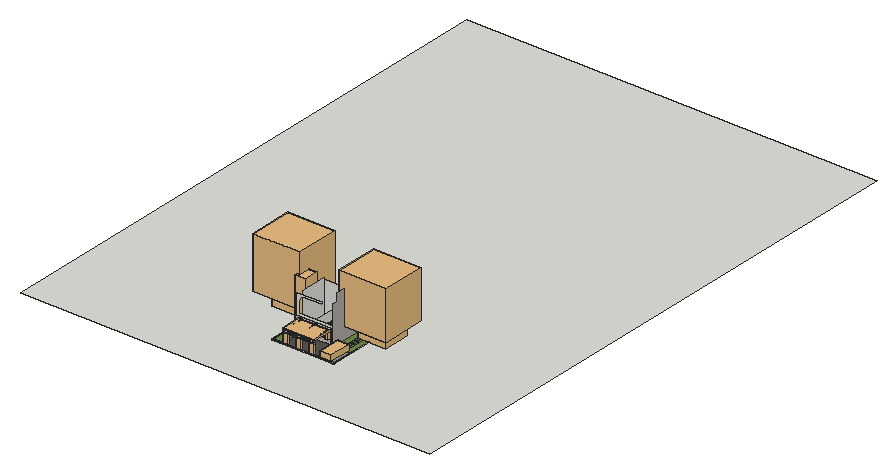
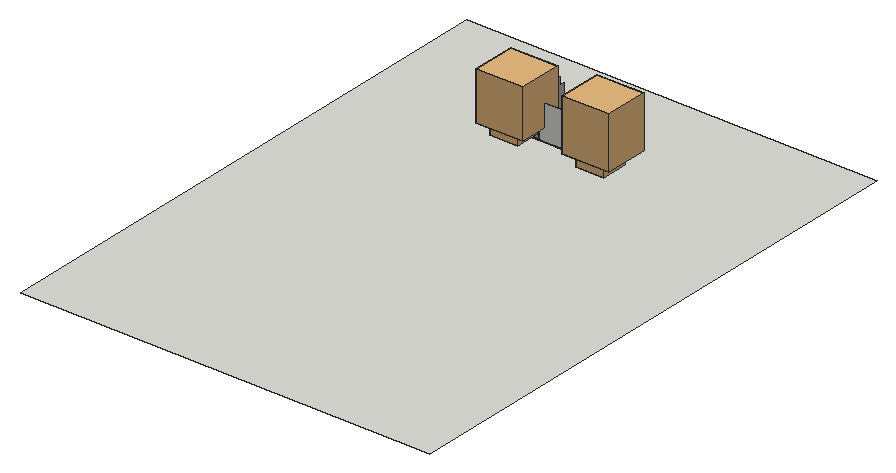
# SketchUp Ruby script. Lengths in inches.
U = 1.inch
M = Sketchup.active_model
def pt(a) = Geom::Point3d.new(a.map { |v| v * U })
def face(e, loops, mat)
  f = e.add_face(loops[0].map { |a| pt(a) })
  loops[1..].each { |l| e.add_face(l.map { |a| pt(a) }).erase! }
  f.material = f.back_material = mat if mat
  f
end
# faces: each face lists its corners as indices into pts; further lists are holes
def faces(e, pts, list, mat = nil) = list.each { |f| face(e, (f[0].is_a?(Array) ? f : [f]).map { |l| l.map { |i| pts[i] } }, mat) }
# xy, xz, yz: faces in a plane at the given z, y or x. An outline is a flat list of corners, or four numbers for a rectangle; further outlines are holes
def ring(l) = l.size == 4 ? [[l[0], l[1]], [l[2], l[1]], [l[2], l[3]], [l[0], l[3]]] : l.each_slice(2).to_a
def flat(e, list, mat, &to3) = list.each { |f| face(e, (f[0].is_a?(Array) ? f : [f]).map { |l| ring(l).map { |u, v| to3.(u, v) } }, mat) }
def xy(e, z, list, mat = nil) = flat(e, list, mat) { |x, y| [x, y, z] }
def xz(e, y, list, mat = nil) = flat(e, list, mat) { |x, z| [x, y, z] }
def yz(e, x, list, mat = nil) = flat(e, list, mat) { |y, z| [x, y, z] }
def lines(e, pts, list) = list.each { |a, b| e.add_line(pt(pts[a]), pt(pts[b])) }
# prism: a flat outline (further loops are holes) pulled along v
def prism(e, loops, v, mat = nil)
  f = face(e, loops, mat); d = Geom::Vector3d.new(v.map { |x| x * U })
  f.pushpull(f.normal.samedirection?(d) ? d.length : -d.length)
end
def box(e, o, s, mat = nil) = prism(e, [[o, [o[0] + s[0], o[1], o[2]], [o[0] + s[0], o[1] + s[1], o[2]], [o[0], o[1] + s[1], o[2]]]], [0, 0, s[2]], mat)
def at(x, y, z, deg = 0) = Geom::Transformation.translation(pt([x, y, z])) * Geom::Transformation.rotation(ORIGIN, Z_AXIS, deg.degrees)
def axes(o, x, y, z) = Geom::Transformation.new([*x, 0, *y, 0, *z, 0, *pt(o).to_a, 1])
def part(name) = M.definitions.add(name)
# library, detail: a bought-in or finely detailed component or shape, given as its bounding box
def library(name, o, s) = part(name).tap { |d| box(d.entities, o, s) }
def detail(e, o, s) = box(e.add_group.entities, o, s)
def put(e, d, t, mat = nil) = e.add_instance(d, t).tap { |i| i.material = mat if mat }
def group(e, t, mat = nil) = e.add_group.tap { |g| g.transformation = t; g.material = mat if mat }.entities
root = M.entities
M.materials.add("AM113_062_Tilia").color = [58, 81, 37]
M.materials.add("AM113_062_Tilia_Bark").color = [88, 85, 72]
M.materials.add("Grass D 200cm").color = [112, 140, 73]
M.materials.add("Grass D 200cm\#1").color = [112, 140, 73]
M.materials.add("Pavement Concrete 03 300cm").color = [155, 154, 151]
M.materials.add("Pavement Rock Tiles 19-79 250cm").color = [91, 85, 85]
M.materials.add("Sandstone 150cm").color = [161, 146, 124]
M.materials.add("Stone D 150cm").color = [179, 173, 168]
M.materials.add("Tiles L01 200cm").color = [179, 171, 162]
M.materials.add("Wall Paint Fine Grain 01 Yellow 100cm").color = [244, 233, 200]
M.materials.add("Wood066_2K_Color").color = [89, 51, 19]
M.materials.add("[Color M05]").color = [114, 114, 114]
M.materials.add("[Color M07]1").color = [58, 58, 58]
M.materials.add("[Color M08]").color = [30, 30, 30]
M.materials.add("[Tile_Various_Tan]").color = [214, 196, 169]
c1 = part("Group3\#2")
p = [[646.26,365.625,0],[646.26,367.5625,0],[646.26,485.6875,58.75],[646.26,523.125,58.75],[725.07,523.125,58.75],[725.07,485.6875,58.75],
  [725.07,367.5625,117.5],[725.07,355.75,117.5],[681.76,365.625,0],[681.76,367.5625,0],[681.76,485.6875,58.75],[681.76,487.625,58.75],
  [689.57,487.625,58.75],[689.57,485.6875,58.75],[689.57,367.5625,117.5],[689.57,355.75,117.5]]
lines(c1.entities,p,[[0,1],[1,2],[2,3],[3,4],[4,5],[5,6],[6,7],[8,9],[9,10],[10,11],[11,12],[12,13],
  [13,14],[14,15]])
c2 = part("Group2\#1")
xy(c2.entities,-3.9375,[[644.32,379.375,683.7,380.3]])
xy(c2.entities,0,[[644.32,367.5625,683.7,379.375]])
xy(c2.entities,5.875,[[644.32,379.375,683.7,391.1875]])
xy(c2.entities,11.75,[[644.32,391.1875,683.7,403]])
xy(c2.entities,17.625,[[644.32,403,683.7,414.8125]])
xy(c2.entities,23.5,[[644.32,414.8125,683.7,426.625]])
xy(c2.entities,29.375,[[644.32,426.625,683.7,438.4375]])
xy(c2.entities,35.25,[[644.32,438.4375,683.7,450.25]])
xy(c2.entities,41.125,[[644.32,450.25,683.7,462.0625]])
xy(c2.entities,47,[[644.32,462.0625,683.7,473.875]])
xy(c2.entities,52.875,[[644.32,473.875,683.7,485.6875]])
xy(c2.entities,54.8125,[[687.63,472.95,687.63,485.6875,683.7,485.6875,683.7,498.42,644.32,498.42,644.32,525.0625,727.01,525.0625,727.01,472.95]])
xy(c2.entities,58.75,[[687.63,473.875,727.01,473.875,727.01,525.0625,644.32,525.0625,644.32,485.6875,687.63,485.6875]])
xy(c2.entities,64.625,[[687.63,462.0625,727.01,473.875]])
xy(c2.entities,70.5,[[687.63,450.25,727.01,462.0625]])
xy(c2.entities,76.375,[[687.63,438.4375,727.01,450.25]])
xy(c2.entities,82.25,[[687.63,426.625,727.01,438.4375]])
xy(c2.entities,88.125,[[687.63,414.8125,727.01,426.625]])
xy(c2.entities,94,[[687.63,403,727.01,414.8125]])
xy(c2.entities,99.875,[[687.63,391.1875,727.01,403]])
xy(c2.entities,105.75,[[687.63,379.375,727.01,391.1875]])
xy(c2.entities,111.625,[[687.63,367.5625,727.01,379.375]])
xy(c2.entities,117.5,[[687.63,355.75,727.01,367.5625]])
xz(c2.entities,367.5625,[[687.63,111.625,727.01,117.5]])
xz(c2.entities,379.375,[[687.63,105.75,727.01,111.625]])
xz(c2.entities,379.375,[[644.32,0,683.7,5.875]],"[Color M05]")
xz(c2.entities,391.1875,[[687.63,99.875,727.01,105.75]])
xz(c2.entities,391.1875,[[644.32,5.875,683.7,11.75]],"[Color M05]")
xz(c2.entities,403,[[687.63,94,727.01,99.875]])
xz(c2.entities,403,[[644.32,11.75,683.7,17.625]],"[Color M05]")
xz(c2.entities,414.8125,[[687.63,88.125,727.01,94]])
xz(c2.entities,414.8125,[[644.32,17.625,683.7,23.5]],"[Color M05]")
xz(c2.entities,426.625,[[687.63,82.25,727.01,88.125]])
xz(c2.entities,426.625,[[644.32,23.5,683.7,29.375]],"[Color M05]")
xz(c2.entities,438.4375,[[687.63,76.375,727.01,82.25]])
xz(c2.entities,438.4375,[[644.32,29.375,683.7,35.25]],"[Color M05]")
xz(c2.entities,450.25,[[687.63,70.5,727.01,76.375]])
xz(c2.entities,450.25,[[644.32,35.25,683.7,41.125]],"[Color M05]")
xz(c2.entities,462.0625,[[687.63,64.625,727.01,70.5]])
xz(c2.entities,462.0625,[[644.32,41.125,683.7,47]],"[Color M05]")
xz(c2.entities,473.875,[[687.63,58.75,727.01,64.625]])
xz(c2.entities,473.875,[[644.32,47,683.7,52.875]],"[Color M05]")
xz(c2.entities,485.6875,[[644.32,52.875,683.7,58.75],[683.7,54.8125,687.63,58.75]],"[Color M05]")
xz(c2.entities,525.0625,[[644.32,54.8125,727.01,58.75]])
yz(c2.entities,644.32,[[379.375,-3.9375,379.375,5.875,391.1875,5.875,391.1875,11.75,403,11.75,403,17.625,414.8125,17.625,414.8125,23.5,426.625,23.5,426.625,29.375,438.4375,29.375,438.4375,35.25,450.25,35.25,450.25,41.125,462.0625,41.125,462.0625,47,473.875,47,473.875,52.875,485.6875,52.875,485.6875,58.75,525.0625,58.75,525.0625,54.8125,498.42,54.8125,380.3,-3.9375]])
yz(c2.entities,683.7,[[379.375,-3.9375,380.3,-3.9375,498.42,54.8125,485.6875,54.8125,485.6875,52.875,473.875,52.875,473.875,47,462.0625,47,462.0625,41.125,450.25,41.125,450.25,35.25,438.4375,35.25,438.4375,29.375,426.625,29.375,426.625,23.5,414.8125,23.5,414.8125,17.625,403,17.625,403,11.75,391.1875,11.75,391.1875,5.875,379.375,5.875]],"[Color M05]")
yz(c2.entities,687.63,[[472.95,54.8125,354.83,113.5625,355.75,113.5625,355.75,117.5,367.5625,117.5,367.5625,111.625,379.375,111.625,379.375,105.75,391.1875,105.75,391.1875,99.875,403,99.875,403,94,414.8125,94,414.8125,88.125,426.625,88.125,426.625,82.25,438.4375,82.25,438.4375,76.375,450.25,76.375,450.25,70.5,462.0625,70.5,462.0625,64.625,473.875,64.625,473.875,58.75,485.6875,58.75,485.6875,54.8125]],"[Color M05]")
yz(c2.entities,727.01,[[472.95,54.8125,525.0625,54.8125,525.0625,58.75,473.875,58.75,473.875,64.625,462.0625,64.625,462.0625,70.5,450.25,70.5,450.25,76.375,438.4375,76.375,438.4375,82.25,426.625,82.25,426.625,88.125,414.8125,88.125,414.8125,94,403,94,403,99.875,391.1875,99.875,391.1875,105.75,379.375,105.75,379.375,111.625,367.5625,111.625,367.5625,117.5,355.75,117.5,355.75,113.5625,354.83,113.5625]])
p = [[644.32,380.3,-3.9375],[644.32,498.42,54.8125],[683.7,498.42,54.8125],[683.7,380.3,-3.9375],[727.01,472.95,54.8125],[727.01,354.83,113.5625],
  [687.63,354.83,113.5625],[687.63,472.95,54.8125]]
faces(c2.entities,p,[[0,1,2,3]])
faces(c2.entities,p,[[4,5,6,7]],"[Color M05]")
put(c2.entities,c1,at(0,0,39.375))
c3 = library("Car 026",[-43.02,-94.05,-1.1],[86.04,187.94,58.68])
c4 = library("Plant",[-27.84,-31.84,-1.26],[68.28,70.82,154.38])
c5 = library("Agrupar\#1",[0,0,-45.2],[34.59,10.39,63.98])
c6 = library("AM113_062_Tilia_Defintion",[-350.67,-364.73,-2.58],[672.29,726.36,1000])
c7 = library("AM113_062_Tilia_Defintion1",[-524.84,-500,219.37],[933.41,1000,877.77])
c8 = part("Group4\#1")
put(c8.entities,c6,axes([0,0,0],[0.28109,0,0],[0,0.28109,0],[0,0,0.28109]),"AM113_062_Tilia_Bark")
put(c8.entities,c7,axes([0,0,0],[0.33697,0,0],[0,0.33697,0],[0,0,0.33697]),"AM113_062_Tilia")
c9 = library("Group4\#2",[-14.05,-12.91,-0.09],[26.62,27.13,73.11])
c10 = library("Agrupar\#17",[0,0,-45.2],[34.59,10.39,63.98])
c11 = library("Agrupar\#6",[0,0,-45.2],[34.59,10.39,63.98])
c12 = library("Shrub+_Grass",[-121.83,-22.34,0],[123.96,19.94,123.95])
c13 = part("Window (2)")
xy(c13.entities,31.72,[[-0.78,88.6,2.72,128.1]])
xy(c13.entities,34.95,[[-0.78,91.53,0.84,106.59],[0.84,91.53,1.05,97.58],[1.05,91.53,1.42,106.59],[1.42,91.53,2.72,106.59],[0.84,97.58,1.05,98.18],
  [0.84,98.18,1.05,106.59]])
xy(c13.entities,35.27,[[-0.78,110.09,0.97,125.14],[1.05,110.09,2.72,125.14]])
xy(c13.entities,58.35,[[2.72,108.74,3.8,109.74]])
xy(c13.entities,77.8125,[[-0.78,110.09,2.72,125.14],[0.97,110.09,1.05,125.14]])
xy(c13.entities,77.93,[[-0.78,91.53,0.84,106.59],[1.05,91.53,1.42,106.59],[1.42,91.53,2.72,106.59]])
xy(c13.entities,80.72,[[-0.78,88.6,2.72,128.1]])
xz(c13.entities,88.6,[[-0.78,31.72,2.72,80.72]])
xz(c13.entities,91.53,[[-0.78,34.95,0.84,77.93],[1.05,34.95,1.42,77.93],[1.42,34.95,2.72,77.93]])
xz(c13.entities,106.59,[[-0.78,34.95,0.84,77.93],[0.84,34.95,1.05,77.93],[0.84,34.95,2.72,77.93]])
xz(c13.entities,108.74,[[3.8,54.35,4.22,54.6,4.22,59.47,2.72,59.97,2.72,58.35,3.8,58.35]])
xz(c13.entities,109.74,[[3.8,54.35,3.8,58.35,2.72,58.35,2.72,59.97,4.22,59.47,4.22,54.6]])
xz(c13.entities,110.09,[[-0.78,35.27,0.97,77.8125],[1.05,35.27,2.72,77.8125]])
xz(c13.entities,125.14,[[-0.78,35.27,0.97,77.8125],[0.97,35.27,1.05,80.72],[1.05,35.27,2.72,77.8125]])
xz(c13.entities,128.1,[[-0.78,31.72,2.72,80.72]])
yz(c13.entities,-0.78,[[[88.6,31.72,128.1,80.72],[91.53,34.95,106.59,77.93],[110.09,35.27,125.14,77.8125]]])
yz(c13.entities,0.84,[[91.53,34.95,106.59,77.93]])
yz(c13.entities,0.97,[[110.09,35.27,125.14,77.8125]])
yz(c13.entities,1.05,[[91.53,34.95,106.59,77.93],[110.09,35.27,125.14,77.8125]])
yz(c13.entities,1.42,[[91.53,34.95,106.59,77.93]])
yz(c13.entities,2.72,[[[88.6,31.72,108.35,80.72],[91.53,34.95,106.59,77.93]],[[108.35,31.72,128.1,80.72],[110.09,35.27,125.14,77.8125],[108.74,58.35,109.74,59.97]]])
yz(c13.entities,3.8,[[108.74,54.35,109.74,58.35]])
yz(c13.entities,4.22,[[108.74,54.6,109.74,59.47]])
p = [[4.22,108.74,54.6],[3.8,108.74,54.35],[3.8,109.74,54.35],[4.22,109.74,54.6],[2.72,109.74,59.97],[2.72,108.74,59.97],
  [4.22,108.74,59.47],[4.22,109.74,59.47],[-0.78,86.4,89.94],[-0.78,86.44,89.94],[15.22,130.69,89.94],[15.22,130.65,89.94],
  [-0.78,86.44,28.19],[-0.78,86.4,28.19],[7.72,130.69,89.94],[7.72,130.65,89.94]]
faces(c13.entities,p,[[0,1,2,3],[4,5,6,7]])
lines(c13.entities,p,[[8,9],[10,11],[12,13],[14,15]])
c14 = library("Plant\#1",[-21.8,-11.875,0],[94.69,106.42,111.78])
c15 = part("Agrupar\#9")
prism(c15.entities,[[[223.78,9.67,1.43],[223.78,1.8,1.43],[-4.57,1.8,1.21],[-4.57,9.67,1.21]]],[-0.01,0,5.85])
p = [[218.86,1.8,0],[218.86,1.8,1.4],[218.86,9.68,1.4],[9.21,0.03,7.27],[9.18,0.03,7.27],[210,0,7.27],
  [209.97,0,7.27],[218.86,1.8,1.42],[9.21,0.03,7.27],[9.21,0,7.27],[210,9.67,1.4],[210,0.03,7.27],
  [209.97,0.03,7.27]]
lines(c15.entities,p,[[0,1],[1,2],[3,4],[5,6],[7,1],[8,9],[2,10],[11,5],[6,12],[12,11]])
c16 = part("Agrupar\#15")
prism(c16.entities,[[[7.43,175.26,4.98],[7.43,0,0],[7.43,0,13.77],[7.43,175.26,18.73]]],[-4.96,0,0])
p = [[3.57,19.55,0.34],[0.01,19.55,0.33],[0,11.68,0.33],[9.92,11.68,0.34]]
lines(c16.entities,p,[[0,1],[2,3]])
c17 = part("Agrupar\#11")
prism(c17.entities,[[[2.47,0,0],[2.47,175.26,4.98],[2.47,175.26,18.73],[2.47,0,13.77]]],[4.96,0,0])
p = [[3.57,19.55,0.34],[0.01,19.55,0.33],[6.3,204.91,6.81],[6.32,204.91,6.81],[0,11.68,0.33],[9.92,11.68,0.34]]
lines(c17.entities,p,[[0,1],[2,3],[4,5]])
c18 = library("Lugstar Premium LED 152 063",[-3.77,-3.75,-3.3125],[7.54,7.53,3.3125])
c19 = part("Tlon Cubo 860 Ceiling 152 005")
xy(c19.entities,-3.04,[[-16.54,-16.54,-16.54,16.54,16.54,-16.54],[16.54,-16.54,-16.54,16.54,16.54,16.54]])
xy(c19.entities,0,[[-16.93,-16.93,16.93,-16.93,-16.93,16.93],[16.93,-16.93,16.93,16.93,-16.93,16.93]])
xz(c19.entities,-16.93,[[-16.93,-3.79,16.93,-3.79,-16.93,0],[16.93,-3.79,16.93,0,-16.93,0]])
xz(c19.entities,-16.3,[[-16.3,-3.66,-16.3,-3.24,16.3,-3.24],[-16.3,-3.66,16.3,-3.24,16.3,-3.66]])
xz(c19.entities,16.3,[[-16.3,-3.66,16.3,-3.24,-16.3,-3.24],[-16.3,-3.66,16.3,-3.66,16.3,-3.24]])
xz(c19.entities,16.93,[[-16.93,-3.79,-16.93,0,16.93,0],[-16.93,-3.79,16.93,0,16.93,-3.79]])
yz(c19.entities,-16.93,[[-16.93,-3.79,-16.93,0,16.93,0],[-16.93,-3.79,16.93,0,16.93,-3.79]])
yz(c19.entities,-16.3,[[-16.3,-3.66,16.3,-3.66,-16.3,-3.24],[16.3,-3.66,16.3,-3.24,-16.3,-3.24]])
yz(c19.entities,16.3,[[-16.3,-3.66,-16.3,-3.24,16.3,-3.66],[16.3,-3.66,-16.3,-3.24,16.3,-3.24]])
yz(c19.entities,16.93,[[-16.93,-3.79,16.93,-3.79,-16.93,0],[16.93,-3.79,16.93,0,-16.93,0]])
p = [[-16.93,-16.93,-3.79],[-16.93,16.93,-3.79],[-16.3,16.3,-3.66],[-16.3,-16.3,-3.66],[16.93,-16.93,-3.79],[16.3,-16.3,-3.66],
  [16.93,16.93,-3.79],[16.3,16.3,-3.66]]
faces(c19.entities,p,[[0,1,2],[2,3,0],[4,0,3],[3,5,4],[6,4,5],[5,7,6],[2,1,6],[6,7,2]])
c20 = library("Agrupar\#14",[0,0,0],[228.36,164.44,7.63])
xy(root,-4.58,[[0,0,3194.52,4346.8125]])
xy(root,0,[[1559.33,498.44,1644.4,897.48],[1644.4,498.44,1909.65,897.48],[1909.65,498.44,2046.34,897.48]])
xy(root,2.95,[[1924.62,498.44,2032.54,504.56]])
xy(root,4.83,[[1872.15,498.44,1924.62,504.56],[1888.73,659.65,1909.65,659.65,1909.65,897.48,1644.4,897.48,1644.4,661.93,1678.32,661.93,1678.32,661.04,1681.48,661.04,1681.48,661.93,1728.89,661.93,1728.89,661.04,1732.04,661.04,1732.04,661.93,1766.5625,661.93,1766.5625,864.08,1892.58,864.08,1892.58,678.73,1888.73,678.73]])
xy(root,4.83,[[1568.1,509.63,1644.4,892.47]],"Grass D 200cm")
xy(root,4.83,[[1909.65,659.65,1960.04,659.65,1960.04,889.59,2002.48,889.59,2002.48,659.65,2039.91,659.65,2039.91,891.36,1909.65,891.36],[[1960.04,659.65,2002.48,889.59],[1963.95,709,1998.57,727.33],[1964.1,760.22,1998.42,778.1],[1963.83,683.72,1998.69,701.3],[1964.62,786.73,1997.91,805.03],[1964.8125,814.375,1997.71,832.89],[1965.02,842.65,1997.5,861.09],[1964.08,735.28,1998.44,752.125],[1965.63,868.98,1996.9,885.96],[1963.49,663.1,1999.03,676.48]]],"Grass D 200cm\#1")
xy(root,4.83,[[1909.65,504.56,2039.91,659.65]],"Pavement Concrete 03 300cm")
xy(root,4.83,[[1644.4,498.44,1872.15,498.44,1872.15,504.56,1909.65,504.56,1909.65,659.65,1888.73,659.65,1888.73,661.93,1732.04,661.93,1732.04,661.04,1728.89,661.04,1728.89,661.93,1681.48,661.93,1681.48,661.04,1678.32,661.04,1678.32,661.93,1644.4,661.93]],"Pavement Rock Tiles 19-79 250cm")
xy(root,4.83,[[1963.49,663.1,1999.03,676.48],[1963.83,683.72,1998.69,701.3],[1963.95,709,1998.57,727.33],[1964.08,735.28,1998.44,752.125],[1964.1,760.22,1998.42,778.1],
  [1964.62,786.73,1997.91,805.03],[1964.8125,814.375,1997.71,832.89],[1965.02,842.65,1997.5,861.09],[1965.63,868.98,1996.9,885.96]],"Sandstone 150cm")
xy(root,4.83,[[1766.5625,661.93,1888.73,661.93,1888.73,678.73,1892.58,678.73,1892.58,864.08,1766.5625,864.08]],"Tiles L01 200cm")
xy(root,4.83,[[1559.33,498.44,1644.4,498.44,1644.4,509.63,1568.1,509.63,1568.1,892.47,1644.4,892.47,1644.4,897.48,1559.33,897.48],[2032.54,498.44,2046.34,498.44,2046.34,897.48,1909.65,897.48,1909.65,891.36,2039.91,891.36,2039.91,504.56,2032.54,504.56]],"Wall Paint Fine Grain 01 Yellow 100cm")
xy(root,21.34,[[1732.04,661.04,1766.5625,661.93]],"[Color M08]")
xy(root,21.51,[[1643.15,661.04,1643.15,701.28,1644.4,701.28,1644.4,661.93,1678.32,661.93,1678.32,661.04]],"[Color M08]")
xy(root,23.78,[[1643.15,661.04,1678.32,661.04,1678.32,661.93,1644.4,661.93,1644.4,701.28,1643.15,701.28],[1732.04,661.04,1766.5625,661.93]],"[Color M08]")
xy(root,38.75,[[1681.48,661.04,1728.89,661.93]],"[Color M08]")
xy(root,41.27,[[1681.48,661.04,1728.89,692.9]])
xy(root,82.25,[[1681.48,661.04,1728.89,692.9]])
xy(root,84.58,[[1681.48,661.04,1728.89,661.93]],"[Color M08]")
xy(root,97.94,[[1766.5625,667.76,1888.73,675.17]])
xy(root,102.9,[[1643.34,661.04,1643.34,701.28,1644.4,701.28,1644.4,661.93,1678.32,661.93,1678.32,661.04]],"[Color M07]1")
xy(root,102.9,[[1681.48,661.04,1728.89,661.93],[1732.04,661.04,1766.5625,661.93]],"[Color M08]")
xz(root,492.91,[[1661.45,86.34,1666.72,102.49]])
xz(root,498.44,[[1559.33,0,1644.4,4.83],[1644.4,0,2046.34,0,2046.34,4.83,2032.54,4.83,2032.54,2.95,1924.62,2.95,1924.62,4.83,1644.4,4.83]],"Wall Paint Fine Grain 01 Yellow 100cm")
xz(root,504.56,[[1924.62,2.95,2032.54,4.83]])
xz(root,654.85,[[[1661.45,92.1875,1666.72,108.31],[1662.42,93.39,1665.64,95.11]],[1662.42,93.39,1665.64,95.11]])
xz(root,659.65,[[1888.73,4.83,1909.65,4.83,1909.65,146.4,1646.56,146.4,1646.56,227.63,1646.79,232.11,1647.5,236.53,1648.67,240.86,1650.29,245.05,1652.34,249.03,1654.8,252.78,1657.64,256.25,1660.83,259.4,1664.34,262.2,1668.12,264.61,1672.13,266.61,1676.34,268.18,1822.65,268.18,1822.65,283.33,1630.85,283.33,1630.85,126.94,1888.73,126.94]])
xz(root,661.04,[[[1678.32,4.83,1681.48,4.83,1681.48,38.75,1728.89,38.75,1728.89,4.83,1732.04,4.83,1732.04,102.9,1766.5625,102.9,1766.5625,106.05,1643.34,106.05,1643.34,102.9,1678.32,102.9],[1681.48,41.27,1728.89,82.25],[1681.48,84.58,1728.89,102.9]],[1732.04,21.34,1766.5625,23.78],[1643.15,21.51,1678.32,23.78]],"[Color M08]")
xz(root,661.93,[[1644.4,4.83,1678.32,21.51],[1732.04,4.83,1766.5625,21.34],[1644.4,23.78,1678.32,102.9],[1732.04,23.78,1766.5625,102.9]])
xz(root,661.93,[[1681.48,4.83,1728.89,38.75],[1681.48,84.58,1728.89,102.9]],"Wood066_2K_Color")
xz(root,667.76,[[1766.5625,97.94,1888.73,126.94]])
xz(root,675.17,[[1766.5625,97.94,1888.73,135.03]])
xz(root,678.73,[[1888.73,4.83,1892.58,135.03]])
xz(root,692.9,[[1681.48,41.27,1728.89,82.25]])
xz(root,701.28,[[1643.15,21.51,1644.4,23.78],[1643.34,102.9,1644.4,106.05]])
xz(root,864.08,[[1766.5625,4.83,1892.58,135.03]])
xz(root,897.48,[[1559.33,0,1644.4,4.83],[1644.4,0,1909.65,4.83],[1909.65,0,2046.34,4.83],[1644.4,4.83,1909.65,276.43]])
yz(root,1559.33,[[498.44,0,897.48,4.83]])
yz(root,1643.15,[[661.04,21.51,701.28,23.78]],"[Color M08]")
yz(root,1643.34,[[661.04,102.9,701.28,106.05]],"[Color M08]")
yz(root,1644.4,[[498.44,0,897.48,4.83],[661.93,4.83,701.28,21.51],[701.28,4.83,897.48,283.33],[661.93,23.78,701.28,102.9]])
yz(root,1661.45,[[492.91,86.34,654.85,92.1875,654.85,108.31,603.7,106.47,501.15,102.78,492.91,102.49]])
yz(root,1666.72,[[492.91,86.34,492.91,102.49,654.85,108.31,654.85,92.1875]])
yz(root,1678.32,[[661.04,4.83,661.93,21.51]])
yz(root,1678.32,[[661.04,23.78,661.93,102.9]],"[Color M08]")
yz(root,1681.48,[[661.04,4.83,661.93,21.05],[661.04,21.05,661.93,38.75],[661.04,41.27,692.9,82.25],[661.04,84.58,661.93,102.9]])
yz(root,1728.89,[[661.04,41.27,692.9,82.25]])
yz(root,1728.89,[[661.04,4.83,661.93,38.75],[661.04,84.58,661.93,102.9]],"[Color M08]")
yz(root,1732.04,[[661.04,4.83,661.93,21.34],[661.04,23.78,661.93,102.9]])
yz(root,1766.5625,[[661.93,4.83,864.08,4.83,864.08,135.03,675.17,135.03,675.17,97.94,667.76,97.94,667.76,106.05,661.04,106.05,661.04,102.9,661.93,102.9,661.93,23.78,661.04,23.78,661.04,21.34,661.93,21.34]])
yz(root,1888.73,[[659.65,4.83,659.65,126.94,667.76,126.94,667.76,97.94,675.17,97.94,675.17,135.03,678.73,135.03,678.73,4.83]])
yz(root,1892.58,[[678.73,4.83,864.08,135.03]])
yz(root,1909.65,[[659.65,4.83,897.48,4.83,897.48,298.4,852.47,298.4,852.47,357.74,701.34,357.74,701.34,298.4,661.93,298.4,661.93,146.4,659.65,146.4]],"Stone D 150cm")
yz(root,1924.62,[[498.44,2.95,504.56,4.83]])
yz(root,2032.54,[[498.44,2.95,504.56,4.83]])
yz(root,2046.34,[[498.44,0,897.48,4.83]],"Wall Paint Fine Grain 01 Yellow 100cm")
p = [[1661.45,492.91,86.34],[1666.72,492.91,86.34],[1666.72,654.85,92.1875],[1661.45,654.85,92.1875],[1661.45,654.85,108.31],[1666.72,654.85,108.31],
  [1666.72,492.91,102.49],[1661.45,492.91,102.49],[1661.45,501.15,102.78],[1661.45,603.7,106.47],[1661.42,603.7,106.47],[1867.8,508.77,103.06],
  [1867.8,654.85,108.31],[1662.62,510.97,86.74],[1658.83,510.97,86.73],[1658.82,503.71,86.73],[1669.37,503.71,86.74]]
faces(root,p,[[0,1,2,3],[4,5,6,7,8,9]])
lines(root,p,[[10,7],[11,12],[13,14],[15,16]])
put(root,c2,axes([776.54,344.3125,4.83],[1.53654,0,0],[0,0.99145,0],[0,0,0.98387]))
put(root,c3,axes([1970.93,593.375,4.54],[1,0,0],[0,0.91,0],[0,0,0.74]))
put(root,c4,axes([1820.09,714.82,4.83],[0.45045,0,0],[0,0.385,0],[0,0,0.385]))
put(root,c5,axes([1645.52,502.54,57.83],[1.06337,0,0],[0,0.924,0],[0,0,1.17276]),"[Tile_Various_Tan]")
put(root,c8,axes([1419.17,918.12,5.8125],[1.16,0,0],[0,1,0],[0,0,1.36254]))
put(root,c9,axes([1603.58,773.99,5.25],[3.24614,0,0],[0,4.0095,0],[0,0,4.78]))
put(root,c8,axes([2076.04,936.5625,5.75],[1.16,0,0],[0,1,0],[0,0,1.27]))
put(root,c10,axes([1846.5625,502.54,58.04],[1.06337,0,0],[0,0.924,0],[0,0,1.17276]),"[Tile_Various_Tan]")
put(root,c11,axes([1746.29,502.54,58.05],[1.06337,0,0],[0,0.924,0],[0,0,1.17276]),"[Tile_Various_Tan]")
put(root,c12,axes([1758.48,663.45,21.86],[0.73735,0,0],[0,0.88766,0],[0,0,0.67568]))
put(root,c13,axes([1833.73,661.34,14.92],[0,0.385,0],[-1.18396,0,0],[0,0,0.83252]))
put(root,c14,axes([1765.5,832.29,69.97],[0.385,0,0],[0,0.385,0],[0,0,0.385]))
put(root,c15,axes([1648.77,502.04,78.43],[1.06337,0,0],[0,0.924,0],[0,0,1.17276]),"[Tile_Various_Tan]")
put(root,c16,axes([1760.18,492.91,86.34],[1.06337,0,0],[0,0.924,0],[0,0,1.17276]),"[Tile_Various_Tan]")
put(root,c17,axes([1859.9,492.91,86.34],[1.06337,0,0],[0,0.924,0],[0,0,1.17276]),"[Tile_Various_Tan]")
put(root,c18,axes([1846.74,671.06,97.94],[0.95273,0,0],[0,0.87991,0],[0,0,0.76039]))
put(root,c18,axes([1792.24,671.06,97.94],[0.95273,0,0],[0,0.87991,0],[0,0,0.76039]))
put(root,c19,axes([1823.5,671.46,97.94],[0.5,0,0],[0,0.21885,0],[0,0,0.5]))
put(root,c20,axes([1643.92,501.15,102.78],[1.06337,0,0],[0,0.924,0],[0,0,1.17276]))
